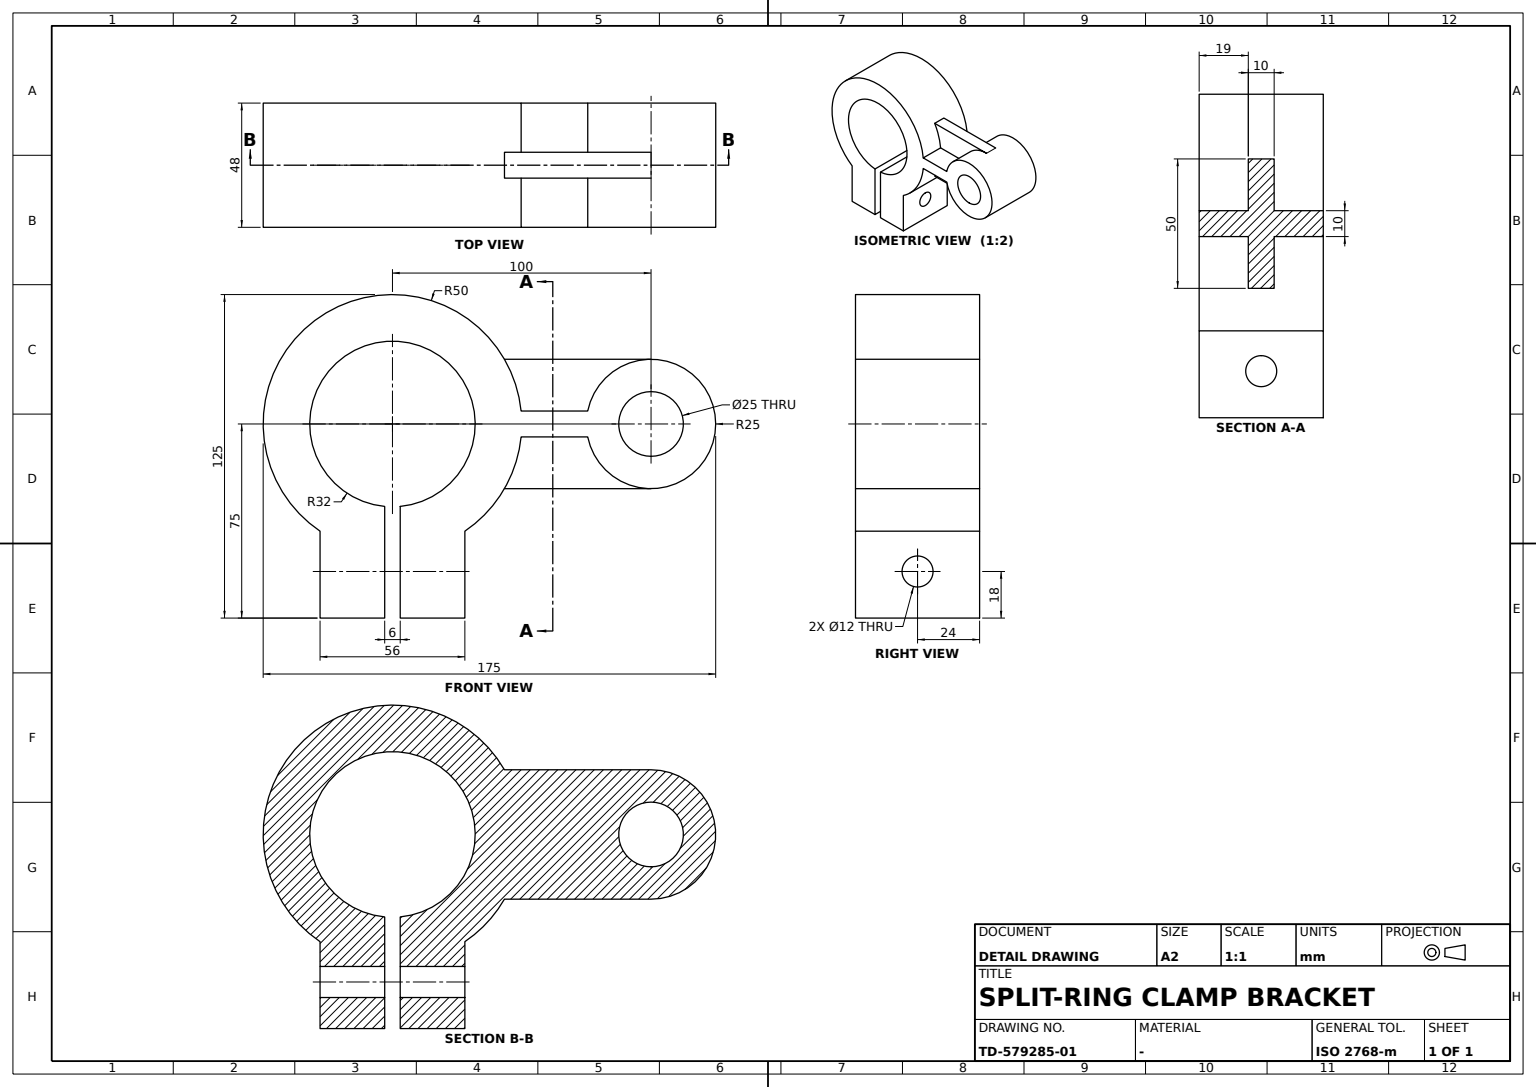
ISO-10303-21;
HEADER;
FILE_DESCRIPTION((''),'2;1');
FILE_NAME('','',(''),(''),'','','');
FILE_SCHEMA(('AUTOMOTIVE_DESIGN'));
ENDSEC;
DATA;
#1=APPLICATION_CONTEXT('');
#2=PRODUCT_CONTEXT('',#1,'mechanical');
#3=PRODUCT('','','',(#2));
#4=PRODUCT_DEFINITION_FORMATION('','',#3);
#5=PRODUCT_DEFINITION_CONTEXT('',#1,'design');
#6=PRODUCT_DEFINITION('','',#4,#5);
#7=PRODUCT_DEFINITION_SHAPE('','',#6);
#8=(LENGTH_UNIT()NAMED_UNIT(*)SI_UNIT(.MILLI.,.METRE.));
#9=(NAMED_UNIT(*)PLANE_ANGLE_UNIT()SI_UNIT($,.RADIAN.));
#10=(NAMED_UNIT(*)SI_UNIT($,.STERADIAN.)SOLID_ANGLE_UNIT());
#11=UNCERTAINTY_MEASURE_WITH_UNIT(LENGTH_MEASURE(0.005),#8,'distance_accuracy_value','');
#12=(GEOMETRIC_REPRESENTATION_CONTEXT(3)GLOBAL_UNCERTAINTY_ASSIGNED_CONTEXT((#11))GLOBAL_UNIT_ASSIGNED_CONTEXT((#8,#9,#10))REPRESENTATION_CONTEXT('',''));
#13=CARTESIAN_POINT('',(-5.,43.30127,25.));
#14=VERTEX_POINT('',#13);
#15=CARTESIAN_POINT('',(-5.,100.,25.));
#16=VERTEX_POINT('',#15);
#17=CARTESIAN_POINT('',(-5.,0.,25.));
#18=DIRECTION('',(0.,1.,0.));
#19=VECTOR('',#18,1000.);
#20=LINE('',#17,#19);
#21=EDGE_CURVE('',#14,#16,#20,.T.);
#22=ORIENTED_EDGE('',*,*,#21,.F.);
#23=CARTESIAN_POINT('',(5.,43.30127,25.));
#24=VERTEX_POINT('',#23);
#25=DIRECTION('',(1.,0.,0.));
#26=VECTOR('',#25,1000.);
#27=LINE('',#13,#26);
#28=EDGE_CURVE('',#14,#24,#27,.T.);
#29=ORIENTED_EDGE('',*,*,#28,.T.);
#30=CARTESIAN_POINT('',(5.,100.,25.));
#31=VERTEX_POINT('',#30);
#32=CARTESIAN_POINT('',(5.,0.,25.));
#33=LINE('',#32,#19);
#34=EDGE_CURVE('',#24,#31,#33,.T.);
#35=ORIENTED_EDGE('',*,*,#34,.T.);
#36=CARTESIAN_POINT('',(0.,100.,25.));
#37=LINE('',#36,#26);
#38=EDGE_CURVE('',#16,#31,#37,.T.);
#39=ORIENTED_EDGE('',*,*,#38,.F.);
#40=EDGE_LOOP('',(#22,#29,#35,#39));
#41=FACE_BOUND('',#40,.T.);
#42=CARTESIAN_POINT('',(0.,43.30127,25.));
#43=DIRECTION('',(0.,0.,-1.));
#44=AXIS2_PLACEMENT_3D('',#42,#43,#18);
#45=PLANE('',#44);
#46=ADVANCED_FACE('',(#41),#45,.F.);
#47=CARTESIAN_POINT('',(-24.,75.505103,-5.));
#48=VERTEX_POINT('',#47);
#49=CARTESIAN_POINT('',(-5.,75.505103,-5.));
#50=VERTEX_POINT('',#49);
#51=LINE('',#47,#26);
#52=EDGE_CURVE('',#48,#50,#51,.T.);
#53=ORIENTED_EDGE('',*,*,#52,.T.);
#54=CARTESIAN_POINT('',(-5.,49.749372,-5.));
#55=VERTEX_POINT('',#54);
#56=CARTESIAN_POINT('',(-5.,0.,-5.));
#57=LINE('',#56,#19);
#58=EDGE_CURVE('',#55,#50,#57,.T.);
#59=ORIENTED_EDGE('',*,*,#58,.F.);
#60=CARTESIAN_POINT('',(-24.,49.749372,-5.));
#61=VERTEX_POINT('',#60);
#62=LINE('',#60,#26);
#63=EDGE_CURVE('',#61,#55,#62,.T.);
#64=ORIENTED_EDGE('',*,*,#63,.F.);
#65=CARTESIAN_POINT('',(-24.,0.,-5.));
#66=LINE('',#65,#19);
#67=EDGE_CURVE('',#61,#48,#66,.T.);
#68=ORIENTED_EDGE('',*,*,#67,.T.);
#69=EDGE_LOOP('',(#53,#59,#64,#68));
#70=FACE_BOUND('',#69,.T.);
#71=CARTESIAN_POINT('',(0.,49.749372,-5.));
#72=AXIS2_PLACEMENT_3D('',#71,#43,#18);
#73=PLANE('',#72);
#74=ADVANCED_FACE('',(#70),#73,.T.);
#75=CARTESIAN_POINT('',(-5.,75.505103,5.));
#76=VERTEX_POINT('',#75);
#77=CARTESIAN_POINT('',(-5.,49.749372,5.));
#78=VERTEX_POINT('',#77);
#79=DIRECTION('',(0.,-1.,0.));
#80=VECTOR('',#79,1000.);
#81=LINE('',#77,#80);
#82=EDGE_CURVE('',#76,#78,#81,.T.);
#83=ORIENTED_EDGE('',*,*,#82,.F.);
#84=CARTESIAN_POINT('',(-24.,75.505103,5.));
#85=VERTEX_POINT('',#84);
#86=LINE('',#84,#26);
#87=EDGE_CURVE('',#85,#76,#86,.T.);
#88=ORIENTED_EDGE('',*,*,#87,.F.);
#89=CARTESIAN_POINT('',(-24.,49.749372,5.));
#90=VERTEX_POINT('',#89);
#91=CARTESIAN_POINT('',(-24.,0.,5.));
#92=LINE('',#91,#19);
#93=EDGE_CURVE('',#90,#85,#92,.T.);
#94=ORIENTED_EDGE('',*,*,#93,.F.);
#95=LINE('',#89,#26);
#96=EDGE_CURVE('',#90,#78,#95,.T.);
#97=ORIENTED_EDGE('',*,*,#96,.T.);
#98=EDGE_LOOP('',(#83,#88,#94,#97));
#99=FACE_BOUND('',#98,.T.);
#100=CARTESIAN_POINT('',(0.,49.749372,5.));
#101=AXIS2_PLACEMENT_3D('',#100,#43,#18);
#102=PLANE('',#101);
#103=ADVANCED_FACE('',(#99),#102,.F.);
#104=CARTESIAN_POINT('',(-24.,-3.,-75.));
#105=VERTEX_POINT('',#104);
#106=CARTESIAN_POINT('',(24.,-3.,-75.));
#107=VERTEX_POINT('',#106);
#108=CARTESIAN_POINT('',(0.,-3.,-75.));
#109=LINE('',#108,#26);
#110=EDGE_CURVE('',#105,#107,#109,.T.);
#111=ORIENTED_EDGE('',*,*,#110,.F.);
#112=CARTESIAN_POINT('',(-24.,-3.,-31.859065));
#113=VERTEX_POINT('',#112);
#114=CARTESIAN_POINT('',(-24.,-3.,0.));
#115=VECTOR('',#43,1000.);
#116=LINE('',#114,#115);
#117=EDGE_CURVE('',#113,#105,#116,.T.);
#118=ORIENTED_EDGE('',*,*,#117,.F.);
#119=CARTESIAN_POINT('',(24.,-3.,-31.859065));
#120=VERTEX_POINT('',#119);
#121=LINE('',#112,#26);
#122=EDGE_CURVE('',#113,#120,#121,.T.);
#123=ORIENTED_EDGE('',*,*,#122,.T.);
#124=CARTESIAN_POINT('',(24.,-3.,0.));
#125=LINE('',#124,#115);
#126=EDGE_CURVE('',#120,#107,#125,.T.);
#127=ORIENTED_EDGE('',*,*,#126,.T.);
#128=EDGE_LOOP('',(#111,#118,#123,#127));
#129=FACE_BOUND('',#128,.T.);
#130=CARTESIAN_POINT('',(0.,-3.,-63.));
#131=VERTEX_POINT('',#130);
#132=CARTESIAN_POINT('',(0.,-3.,-57.));
#133=AXIS2_PLACEMENT_3D('',#132,#79,#43);
#134=CIRCLE('',#133,6.);
#135=EDGE_CURVE('',#131,#131,#134,.T.);
#136=ORIENTED_EDGE('',*,*,#135,.T.);
#137=EDGE_LOOP('',(#136));
#138=FACE_BOUND('',#137,.T.);
#139=CARTESIAN_POINT('',(0.,-3.,-31.859065));
#140=AXIS2_PLACEMENT_3D('',#139,#79,#43);
#141=PLANE('',#140);
#142=ADVANCED_FACE('',(#129,#138),#141,.F.);
#143=CARTESIAN_POINT('',(-5.,100.,0.));
#144=AXIS2_PLACEMENT_3D('',#143,#25,#43);
#145=CIRCLE('',#144,25.);
#146=EDGE_CURVE('',#16,#76,#145,.T.);
#147=ORIENTED_EDGE('',*,*,#146,.T.);
#148=ORIENTED_EDGE('',*,*,#82,.T.);
#149=CARTESIAN_POINT('',(-5.,0.,0.));
#150=AXIS2_PLACEMENT_3D('',#149,#25,#43);
#151=CIRCLE('',#150,50.);
#152=EDGE_CURVE('',#78,#14,#151,.T.);
#153=ORIENTED_EDGE('',*,*,#152,.T.);
#154=ORIENTED_EDGE('',*,*,#21,.T.);
#155=EDGE_LOOP('',(#147,#148,#153,#154));
#156=FACE_BOUND('',#155,.T.);
#157=AXIS2_PLACEMENT_3D('',#149,#25,#18);
#158=PLANE('',#157);
#159=ADVANCED_FACE('',(#156),#158,.F.);
#160=CARTESIAN_POINT('',(-24.,100.,0.));
#161=AXIS2_PLACEMENT_3D('',#160,#25,#43);
#162=CIRCLE('',#161,25.);
#163=EDGE_CURVE('',#48,#85,#162,.T.);
#164=ORIENTED_EDGE('',*,*,#163,.T.);
#165=ORIENTED_EDGE('',*,*,#87,.T.);
#166=ORIENTED_EDGE('',*,*,#146,.F.);
#167=ORIENTED_EDGE('',*,*,#38,.T.);
#168=CARTESIAN_POINT('',(5.,75.505103,5.));
#169=VERTEX_POINT('',#168);
#170=CARTESIAN_POINT('',(5.,100.,0.));
#171=AXIS2_PLACEMENT_3D('',#170,#25,#43);
#172=CIRCLE('',#171,25.);
#173=EDGE_CURVE('',#31,#169,#172,.T.);
#174=ORIENTED_EDGE('',*,*,#173,.T.);
#175=CARTESIAN_POINT('',(24.,75.505103,5.));
#176=VERTEX_POINT('',#175);
#177=LINE('',#168,#26);
#178=EDGE_CURVE('',#169,#176,#177,.T.);
#179=ORIENTED_EDGE('',*,*,#178,.T.);
#180=CARTESIAN_POINT('',(24.,75.505103,-5.));
#181=VERTEX_POINT('',#180);
#182=CARTESIAN_POINT('',(24.,100.,0.));
#183=AXIS2_PLACEMENT_3D('',#182,#25,#43);
#184=CIRCLE('',#183,25.);
#185=EDGE_CURVE('',#181,#176,#184,.T.);
#186=ORIENTED_EDGE('',*,*,#185,.F.);
#187=CARTESIAN_POINT('',(5.,75.505103,-5.));
#188=VERTEX_POINT('',#187);
#189=LINE('',#187,#26);
#190=EDGE_CURVE('',#188,#181,#189,.T.);
#191=ORIENTED_EDGE('',*,*,#190,.F.);
#192=CARTESIAN_POINT('',(5.,100.,-25.));
#193=VERTEX_POINT('',#192);
#194=EDGE_CURVE('',#188,#193,#172,.T.);
#195=ORIENTED_EDGE('',*,*,#194,.T.);
#196=CARTESIAN_POINT('',(-5.,100.,-25.));
#197=VERTEX_POINT('',#196);
#198=CARTESIAN_POINT('',(0.,100.,-25.));
#199=LINE('',#198,#26);
#200=EDGE_CURVE('',#197,#193,#199,.T.);
#201=ORIENTED_EDGE('',*,*,#200,.F.);
#202=EDGE_CURVE('',#50,#197,#145,.T.);
#203=ORIENTED_EDGE('',*,*,#202,.F.);
#204=ORIENTED_EDGE('',*,*,#52,.F.);
#205=EDGE_LOOP('',(#164,#165,#166,#167,#174,#179,#186,#191,#195,#201,#203,#204));
#206=FACE_BOUND('',#205,.T.);
#207=CARTESIAN_POINT('',(0.,100.,0.));
#208=AXIS2_PLACEMENT_3D('',#207,#25,#18);
#209=CYLINDRICAL_SURFACE('',#208,25.);
#210=ADVANCED_FACE('',(#206),#209,.T.);
#211=CARTESIAN_POINT('',(-24.,3.,-31.859065));
#212=VERTEX_POINT('',#211);
#213=CARTESIAN_POINT('',(-24.,3.,-75.));
#214=VERTEX_POINT('',#213);
#215=CARTESIAN_POINT('',(-24.,3.,0.));
#216=LINE('',#215,#115);
#217=EDGE_CURVE('',#212,#214,#216,.T.);
#218=ORIENTED_EDGE('',*,*,#217,.T.);
#219=CARTESIAN_POINT('',(24.,3.,-75.));
#220=VERTEX_POINT('',#219);
#221=CARTESIAN_POINT('',(0.,3.,-75.));
#222=LINE('',#221,#26);
#223=EDGE_CURVE('',#214,#220,#222,.T.);
#224=ORIENTED_EDGE('',*,*,#223,.T.);
#225=CARTESIAN_POINT('',(24.,3.,-31.859065));
#226=VERTEX_POINT('',#225);
#227=CARTESIAN_POINT('',(24.,3.,0.));
#228=LINE('',#227,#115);
#229=EDGE_CURVE('',#226,#220,#228,.T.);
#230=ORIENTED_EDGE('',*,*,#229,.F.);
#231=LINE('',#211,#26);
#232=EDGE_CURVE('',#212,#226,#231,.T.);
#233=ORIENTED_EDGE('',*,*,#232,.F.);
#234=EDGE_LOOP('',(#218,#224,#230,#233));
#235=FACE_BOUND('',#234,.T.);
#236=CARTESIAN_POINT('',(0.,3.,-63.));
#237=VERTEX_POINT('',#236);
#238=CARTESIAN_POINT('',(0.,3.,-57.));
#239=AXIS2_PLACEMENT_3D('',#238,#79,#43);
#240=CIRCLE('',#239,6.);
#241=EDGE_CURVE('',#237,#237,#240,.T.);
#242=ORIENTED_EDGE('',*,*,#241,.F.);
#243=EDGE_LOOP('',(#242));
#244=FACE_BOUND('',#243,.T.);
#245=CARTESIAN_POINT('',(0.,3.,-31.859065));
#246=AXIS2_PLACEMENT_3D('',#245,#79,#43);
#247=PLANE('',#246);
#248=ADVANCED_FACE('',(#235,#244),#247,.T.);
#249=CARTESIAN_POINT('',(-24.,-28.,-75.));
#250=VERTEX_POINT('',#249);
#251=CARTESIAN_POINT('',(-24.,0.,-75.));
#252=LINE('',#251,#80);
#253=EDGE_CURVE('',#105,#250,#252,.T.);
#254=ORIENTED_EDGE('',*,*,#253,.F.);
#255=ORIENTED_EDGE('',*,*,#110,.T.);
#256=CARTESIAN_POINT('',(24.,-28.,-75.));
#257=VERTEX_POINT('',#256);
#258=CARTESIAN_POINT('',(24.,0.,-75.));
#259=LINE('',#258,#80);
#260=EDGE_CURVE('',#107,#257,#259,.T.);
#261=ORIENTED_EDGE('',*,*,#260,.T.);
#262=CARTESIAN_POINT('',(0.,-28.,-75.));
#263=LINE('',#262,#26);
#264=EDGE_CURVE('',#250,#257,#263,.T.);
#265=ORIENTED_EDGE('',*,*,#264,.F.);
#266=EDGE_LOOP('',(#254,#255,#261,#265));
#267=FACE_BOUND('',#266,.T.);
#268=CARTESIAN_POINT('',(0.,28.,-75.));
#269=DIRECTION('',(0.,0.,1.));
#270=AXIS2_PLACEMENT_3D('',#268,#269,#79);
#271=PLANE('',#270);
#272=ADVANCED_FACE('',(#267),#271,.F.);
#273=CARTESIAN_POINT('',(5.,49.749372,5.));
#274=VERTEX_POINT('',#273);
#275=CARTESIAN_POINT('',(5.,0.,0.));
#276=AXIS2_PLACEMENT_3D('',#275,#25,#43);
#277=CIRCLE('',#276,50.);
#278=EDGE_CURVE('',#274,#24,#277,.T.);
#279=ORIENTED_EDGE('',*,*,#278,.T.);
#280=ORIENTED_EDGE('',*,*,#28,.F.);
#281=ORIENTED_EDGE('',*,*,#152,.F.);
#282=ORIENTED_EDGE('',*,*,#96,.F.);
#283=CARTESIAN_POINT('',(-24.,-28.,-41.42463));
#284=VERTEX_POINT('',#283);
#285=CARTESIAN_POINT('',(-24.,0.,0.));
#286=AXIS2_PLACEMENT_3D('',#285,#25,#43);
#287=CIRCLE('',#286,50.);
#288=EDGE_CURVE('',#90,#284,#287,.T.);
#289=ORIENTED_EDGE('',*,*,#288,.T.);
#290=CARTESIAN_POINT('',(24.,-28.,-41.42463));
#291=VERTEX_POINT('',#290);
#292=LINE('',#283,#26);
#293=EDGE_CURVE('',#284,#291,#292,.T.);
#294=ORIENTED_EDGE('',*,*,#293,.T.);
#295=CARTESIAN_POINT('',(24.,49.749372,5.));
#296=VERTEX_POINT('',#295);
#297=CARTESIAN_POINT('',(24.,0.,0.));
#298=AXIS2_PLACEMENT_3D('',#297,#25,#43);
#299=CIRCLE('',#298,50.);
#300=EDGE_CURVE('',#296,#291,#299,.T.);
#301=ORIENTED_EDGE('',*,*,#300,.F.);
#302=LINE('',#273,#26);
#303=EDGE_CURVE('',#274,#296,#302,.T.);
#304=ORIENTED_EDGE('',*,*,#303,.F.);
#305=EDGE_LOOP('',(#279,#280,#281,#282,#289,#294,#301,#304));
#306=FACE_BOUND('',#305,.T.);
#307=CARTESIAN_POINT('',(0.,0.,0.));
#308=AXIS2_PLACEMENT_3D('',#307,#25,#18);
#309=CYLINDRICAL_SURFACE('',#308,50.);
#310=ADVANCED_FACE('',(#306),#309,.T.);
#311=CARTESIAN_POINT('',(24.,49.749372,-5.));
#312=VERTEX_POINT('',#311);
#313=CARTESIAN_POINT('',(24.,0.,-5.));
#314=LINE('',#313,#19);
#315=EDGE_CURVE('',#312,#181,#314,.T.);
#316=ORIENTED_EDGE('',*,*,#315,.F.);
#317=CARTESIAN_POINT('',(5.,49.749372,-5.));
#318=VERTEX_POINT('',#317);
#319=LINE('',#317,#26);
#320=EDGE_CURVE('',#318,#312,#319,.T.);
#321=ORIENTED_EDGE('',*,*,#320,.F.);
#322=CARTESIAN_POINT('',(5.,0.,-5.));
#323=LINE('',#322,#19);
#324=EDGE_CURVE('',#318,#188,#323,.T.);
#325=ORIENTED_EDGE('',*,*,#324,.T.);
#326=ORIENTED_EDGE('',*,*,#190,.T.);
#327=EDGE_LOOP('',(#316,#321,#325,#326));
#328=FACE_BOUND('',#327,.T.);
#329=ADVANCED_FACE('',(#328),#73,.T.);
#330=ORIENTED_EDGE('',*,*,#293,.F.);
#331=CARTESIAN_POINT('',(-24.,-28.,0.));
#332=LINE('',#331,#115);
#333=EDGE_CURVE('',#284,#250,#332,.T.);
#334=ORIENTED_EDGE('',*,*,#333,.T.);
#335=ORIENTED_EDGE('',*,*,#264,.T.);
#336=CARTESIAN_POINT('',(24.,-28.,0.));
#337=LINE('',#336,#115);
#338=EDGE_CURVE('',#291,#257,#337,.T.);
#339=ORIENTED_EDGE('',*,*,#338,.F.);
#340=EDGE_LOOP('',(#330,#334,#335,#339));
#341=FACE_BOUND('',#340,.T.);
#342=CARTESIAN_POINT('',(0.,-28.,-63.));
#343=VERTEX_POINT('',#342);
#344=CARTESIAN_POINT('',(0.,-28.,-57.));
#345=AXIS2_PLACEMENT_3D('',#344,#79,#43);
#346=CIRCLE('',#345,6.);
#347=EDGE_CURVE('',#343,#343,#346,.T.);
#348=ORIENTED_EDGE('',*,*,#347,.F.);
#349=EDGE_LOOP('',(#348));
#350=FACE_BOUND('',#349,.T.);
#351=CARTESIAN_POINT('',(0.,-28.,-41.42463));
#352=AXIS2_PLACEMENT_3D('',#351,#79,#43);
#353=PLANE('',#352);
#354=ADVANCED_FACE('',(#341,#350),#353,.T.);
#355=CARTESIAN_POINT('',(-24.,100.,-12.5));
#356=VERTEX_POINT('',#355);
#357=CIRCLE('',#161,12.5);
#358=EDGE_CURVE('',#356,#356,#357,.T.);
#359=ORIENTED_EDGE('',*,*,#358,.T.);
#360=EDGE_LOOP('',(#359));
#361=FACE_BOUND('',#360,.T.);
#362=CIRCLE('',#286,32.);
#363=EDGE_CURVE('',#212,#113,#362,.T.);
#364=ORIENTED_EDGE('',*,*,#363,.T.);
#365=ORIENTED_EDGE('',*,*,#117,.T.);
#366=ORIENTED_EDGE('',*,*,#253,.T.);
#367=ORIENTED_EDGE('',*,*,#333,.F.);
#368=ORIENTED_EDGE('',*,*,#288,.F.);
#369=ORIENTED_EDGE('',*,*,#93,.T.);
#370=ORIENTED_EDGE('',*,*,#163,.F.);
#371=ORIENTED_EDGE('',*,*,#67,.F.);
#372=CARTESIAN_POINT('',(-24.,28.,-41.42463));
#373=VERTEX_POINT('',#372);
#374=EDGE_CURVE('',#373,#61,#287,.T.);
#375=ORIENTED_EDGE('',*,*,#374,.F.);
#376=CARTESIAN_POINT('',(-24.,28.,-75.));
#377=VERTEX_POINT('',#376);
#378=CARTESIAN_POINT('',(-24.,28.,0.));
#379=VECTOR('',#269,1000.);
#380=LINE('',#378,#379);
#381=EDGE_CURVE('',#377,#373,#380,.T.);
#382=ORIENTED_EDGE('',*,*,#381,.F.);
#383=EDGE_CURVE('',#377,#214,#252,.T.);
#384=ORIENTED_EDGE('',*,*,#383,.T.);
#385=ORIENTED_EDGE('',*,*,#217,.F.);
#386=EDGE_LOOP('',(#364,#365,#366,#367,#368,#369,#370,#371,#375,#382,#384,#385));
#387=FACE_BOUND('',#386,.T.);
#388=AXIS2_PLACEMENT_3D('',#285,#25,#18);
#389=PLANE('',#388);
#390=ADVANCED_FACE('',(#361,#387),#389,.F.);
#391=CARTESIAN_POINT('',(-5.,43.30127,-25.));
#392=VERTEX_POINT('',#391);
#393=CARTESIAN_POINT('',(5.,43.30127,-25.));
#394=VERTEX_POINT('',#393);
#395=LINE('',#391,#26);
#396=EDGE_CURVE('',#392,#394,#395,.T.);
#397=ORIENTED_EDGE('',*,*,#396,.F.);
#398=CARTESIAN_POINT('',(-5.,0.,-25.));
#399=LINE('',#398,#19);
#400=EDGE_CURVE('',#392,#197,#399,.T.);
#401=ORIENTED_EDGE('',*,*,#400,.T.);
#402=ORIENTED_EDGE('',*,*,#200,.T.);
#403=CARTESIAN_POINT('',(5.,0.,-25.));
#404=LINE('',#403,#19);
#405=EDGE_CURVE('',#394,#193,#404,.T.);
#406=ORIENTED_EDGE('',*,*,#405,.F.);
#407=EDGE_LOOP('',(#397,#401,#402,#406));
#408=FACE_BOUND('',#407,.T.);
#409=CARTESIAN_POINT('',(0.,43.30127,-25.));
#410=AXIS2_PLACEMENT_3D('',#409,#43,#18);
#411=PLANE('',#410);
#412=ADVANCED_FACE('',(#408),#411,.T.);
#413=ORIENTED_EDGE('',*,*,#278,.F.);
#414=LINE('',#273,#80);
#415=EDGE_CURVE('',#169,#274,#414,.T.);
#416=ORIENTED_EDGE('',*,*,#415,.F.);
#417=ORIENTED_EDGE('',*,*,#173,.F.);
#418=ORIENTED_EDGE('',*,*,#34,.F.);
#419=EDGE_LOOP('',(#413,#416,#417,#418));
#420=FACE_BOUND('',#419,.T.);
#421=AXIS2_PLACEMENT_3D('',#275,#25,#18);
#422=PLANE('',#421);
#423=ADVANCED_FACE('',(#420),#422,.T.);
#424=CARTESIAN_POINT('',(0.,28.,-51.));
#425=VERTEX_POINT('',#424);
#426=CARTESIAN_POINT('',(0.,28.,-57.));
#427=AXIS2_PLACEMENT_3D('',#426,#18,#269);
#428=CIRCLE('',#427,6.);
#429=EDGE_CURVE('',#425,#425,#428,.T.);
#430=ORIENTED_EDGE('',*,*,#429,.F.);
#431=EDGE_LOOP('',(#430));
#432=FACE_BOUND('',#431,.T.);
#433=CARTESIAN_POINT('',(24.,28.,-75.));
#434=VERTEX_POINT('',#433);
#435=CARTESIAN_POINT('',(24.,28.,-41.42463));
#436=VERTEX_POINT('',#435);
#437=CARTESIAN_POINT('',(24.,28.,0.));
#438=LINE('',#437,#379);
#439=EDGE_CURVE('',#434,#436,#438,.T.);
#440=ORIENTED_EDGE('',*,*,#439,.F.);
#441=LINE('',#268,#26);
#442=EDGE_CURVE('',#377,#434,#441,.T.);
#443=ORIENTED_EDGE('',*,*,#442,.F.);
#444=ORIENTED_EDGE('',*,*,#381,.T.);
#445=LINE('',#372,#26);
#446=EDGE_CURVE('',#373,#436,#445,.T.);
#447=ORIENTED_EDGE('',*,*,#446,.T.);
#448=EDGE_LOOP('',(#440,#443,#444,#447));
#449=FACE_BOUND('',#448,.T.);
#450=AXIS2_PLACEMENT_3D('',#268,#18,#269);
#451=PLANE('',#450);
#452=ADVANCED_FACE('',(#432,#449),#451,.T.);
#453=EDGE_CURVE('',#434,#220,#259,.T.);
#454=ORIENTED_EDGE('',*,*,#453,.T.);
#455=ORIENTED_EDGE('',*,*,#223,.F.);
#456=ORIENTED_EDGE('',*,*,#383,.F.);
#457=ORIENTED_EDGE('',*,*,#442,.T.);
#458=EDGE_LOOP('',(#454,#455,#456,#457));
#459=FACE_BOUND('',#458,.T.);
#460=ADVANCED_FACE('',(#459),#271,.F.);
#461=CARTESIAN_POINT('',(24.,100.,-12.5));
#462=VERTEX_POINT('',#461);
#463=CIRCLE('',#183,12.5);
#464=EDGE_CURVE('',#462,#462,#463,.T.);
#465=ORIENTED_EDGE('',*,*,#464,.T.);
#466=EDGE_LOOP('',(#465));
#467=FACE_BOUND('',#466,.T.);
#468=ORIENTED_EDGE('',*,*,#358,.F.);
#469=EDGE_LOOP('',(#468));
#470=FACE_BOUND('',#469,.T.);
#471=CYLINDRICAL_SURFACE('',#208,12.5);
#472=ADVANCED_FACE('',(#467,#470),#471,.F.);
#473=EDGE_CURVE('',#392,#55,#151,.T.);
#474=ORIENTED_EDGE('',*,*,#473,.F.);
#475=ORIENTED_EDGE('',*,*,#396,.T.);
#476=EDGE_CURVE('',#394,#318,#277,.T.);
#477=ORIENTED_EDGE('',*,*,#476,.T.);
#478=ORIENTED_EDGE('',*,*,#320,.T.);
#479=EDGE_CURVE('',#436,#312,#299,.T.);
#480=ORIENTED_EDGE('',*,*,#479,.F.);
#481=ORIENTED_EDGE('',*,*,#446,.F.);
#482=ORIENTED_EDGE('',*,*,#374,.T.);
#483=ORIENTED_EDGE('',*,*,#63,.T.);
#484=EDGE_LOOP('',(#474,#475,#477,#478,#480,#481,#482,#483));
#485=FACE_BOUND('',#484,.T.);
#486=ADVANCED_FACE('',(#485),#309,.T.);
#487=ORIENTED_EDGE('',*,*,#241,.T.);
#488=EDGE_LOOP('',(#487));
#489=FACE_BOUND('',#488,.T.);
#490=ORIENTED_EDGE('',*,*,#429,.T.);
#491=EDGE_LOOP('',(#490));
#492=FACE_BOUND('',#491,.T.);
#493=CARTESIAN_POINT('',(0.,0.,-57.));
#494=DIRECTION('',(-1.,0.,0.));
#495=AXIS2_PLACEMENT_3D('',#493,#18,#494);
#496=CYLINDRICAL_SURFACE('',#495,6.);
#497=ADVANCED_FACE('',(#489,#492),#496,.F.);
#498=ORIENTED_EDGE('',*,*,#126,.F.);
#499=CIRCLE('',#298,32.);
#500=EDGE_CURVE('',#226,#120,#499,.T.);
#501=ORIENTED_EDGE('',*,*,#500,.F.);
#502=ORIENTED_EDGE('',*,*,#229,.T.);
#503=ORIENTED_EDGE('',*,*,#453,.F.);
#504=ORIENTED_EDGE('',*,*,#439,.T.);
#505=ORIENTED_EDGE('',*,*,#479,.T.);
#506=ORIENTED_EDGE('',*,*,#315,.T.);
#507=ORIENTED_EDGE('',*,*,#185,.T.);
#508=CARTESIAN_POINT('',(24.,0.,5.));
#509=LINE('',#508,#19);
#510=EDGE_CURVE('',#296,#176,#509,.T.);
#511=ORIENTED_EDGE('',*,*,#510,.F.);
#512=ORIENTED_EDGE('',*,*,#300,.T.);
#513=ORIENTED_EDGE('',*,*,#338,.T.);
#514=ORIENTED_EDGE('',*,*,#260,.F.);
#515=EDGE_LOOP('',(#498,#501,#502,#503,#504,#505,#506,#507,#511,#512,#513,#514));
#516=FACE_BOUND('',#515,.T.);
#517=ORIENTED_EDGE('',*,*,#464,.F.);
#518=EDGE_LOOP('',(#517));
#519=FACE_BOUND('',#518,.T.);
#520=AXIS2_PLACEMENT_3D('',#297,#25,#18);
#521=PLANE('',#520);
#522=ADVANCED_FACE('',(#516,#519),#521,.T.);
#523=ORIENTED_EDGE('',*,*,#324,.F.);
#524=ORIENTED_EDGE('',*,*,#476,.F.);
#525=ORIENTED_EDGE('',*,*,#405,.T.);
#526=ORIENTED_EDGE('',*,*,#194,.F.);
#527=EDGE_LOOP('',(#523,#524,#525,#526));
#528=FACE_BOUND('',#527,.T.);
#529=ADVANCED_FACE('',(#528),#422,.T.);
#530=ORIENTED_EDGE('',*,*,#135,.F.);
#531=EDGE_LOOP('',(#530));
#532=FACE_BOUND('',#531,.T.);
#533=ORIENTED_EDGE('',*,*,#347,.T.);
#534=EDGE_LOOP('',(#533));
#535=FACE_BOUND('',#534,.T.);
#536=ADVANCED_FACE('',(#532,#535),#496,.F.);
#537=ORIENTED_EDGE('',*,*,#122,.F.);
#538=ORIENTED_EDGE('',*,*,#363,.F.);
#539=ORIENTED_EDGE('',*,*,#232,.T.);
#540=ORIENTED_EDGE('',*,*,#500,.T.);
#541=EDGE_LOOP('',(#537,#538,#539,#540));
#542=FACE_BOUND('',#541,.T.);
#543=CYLINDRICAL_SURFACE('',#308,32.);
#544=ADVANCED_FACE('',(#542),#543,.F.);
#545=ORIENTED_EDGE('',*,*,#202,.T.);
#546=ORIENTED_EDGE('',*,*,#400,.F.);
#547=ORIENTED_EDGE('',*,*,#473,.T.);
#548=ORIENTED_EDGE('',*,*,#58,.T.);
#549=EDGE_LOOP('',(#545,#546,#547,#548));
#550=FACE_BOUND('',#549,.T.);
#551=ADVANCED_FACE('',(#550),#158,.F.);
#552=ORIENTED_EDGE('',*,*,#510,.T.);
#553=ORIENTED_EDGE('',*,*,#178,.F.);
#554=ORIENTED_EDGE('',*,*,#415,.T.);
#555=ORIENTED_EDGE('',*,*,#303,.T.);
#556=EDGE_LOOP('',(#552,#553,#554,#555));
#557=FACE_BOUND('',#556,.T.);
#558=ADVANCED_FACE('',(#557),#102,.F.);
#559=CLOSED_SHELL('',(#46,#74,#103,#142,#159,#210,#248,#272,#310,#329,#354,#390,#412,#423,#452,#460,#472,#486,#497,#522,#529,#536,#544,#551,#558));
#560=MANIFOLD_SOLID_BREP('',#559);
#561=ADVANCED_BREP_SHAPE_REPRESENTATION('',(#560),#12);
#562=SHAPE_DEFINITION_REPRESENTATION(#7,#561);
ENDSEC;
END-ISO-10303-21;
